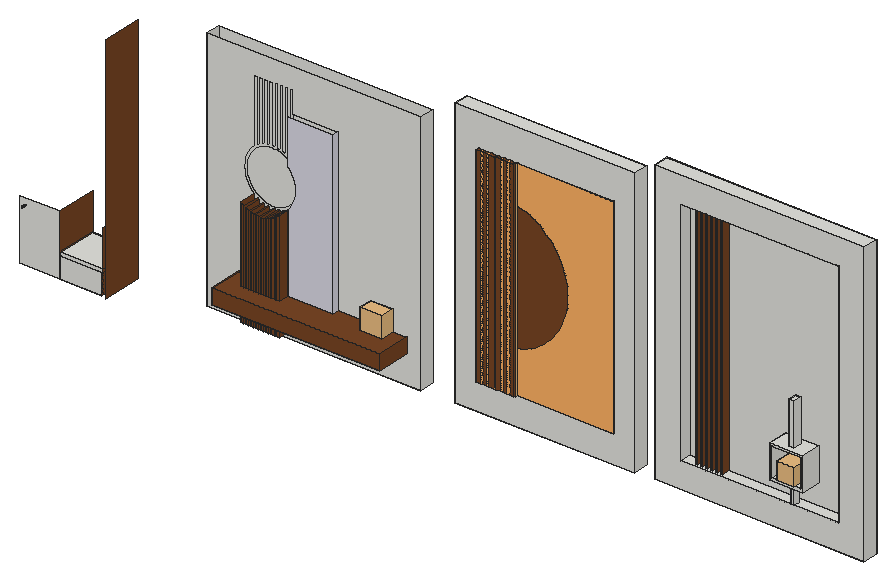
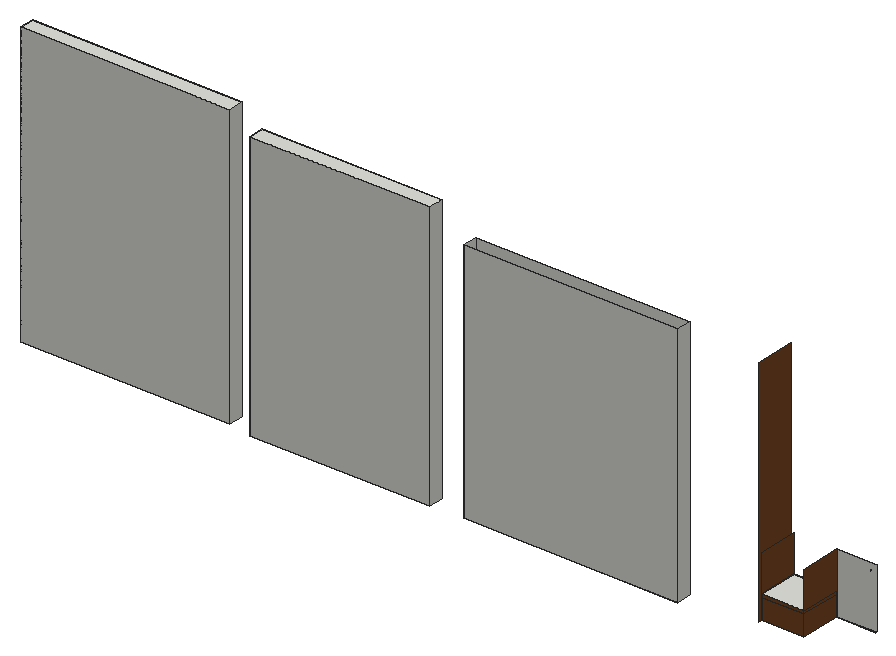
# SketchUp Ruby script. Lengths in inches.
U = 1.inch
M = Sketchup.active_model
def pt(a) = Geom::Point3d.new(a.map { |v| v * U })
def face(e, loops, mat)
  f = e.add_face(loops[0].map { |a| pt(a) })
  loops[1..].each { |l| e.add_face(l.map { |a| pt(a) }).erase! }
  f.material = f.back_material = mat if mat
  f
end
# faces: each face lists its corners as indices into pts; further lists are holes
def faces(e, pts, list, mat = nil) = list.each { |f| face(e, (f[0].is_a?(Array) ? f : [f]).map { |l| l.map { |i| pts[i] } }, mat) }
# xy, xz, yz: faces in a plane at the given z, y or x. An outline is a flat list of corners, or four numbers for a rectangle; further outlines are holes
def ring(l) = l.size == 4 ? [[l[0], l[1]], [l[2], l[1]], [l[2], l[3]], [l[0], l[3]]] : l.each_slice(2).to_a
def flat(e, list, mat, &to3) = list.each { |f| face(e, (f[0].is_a?(Array) ? f : [f]).map { |l| ring(l).map { |u, v| to3.(u, v) } }, mat) }
def xy(e, z, list, mat = nil) = flat(e, list, mat) { |x, y| [x, y, z] }
def xz(e, y, list, mat = nil) = flat(e, list, mat) { |x, z| [x, y, z] }
def yz(e, x, list, mat = nil) = flat(e, list, mat) { |y, z| [x, y, z] }
def lines(e, pts, list) = list.each { |a, b| e.add_line(pt(pts[a]), pt(pts[b])) }
# prism: a flat outline (further loops are holes) pulled along v
def prism(e, loops, v, mat = nil)
  f = face(e, loops, mat); d = Geom::Vector3d.new(v.map { |x| x * U })
  f.pushpull(f.normal.samedirection?(d) ? d.length : -d.length)
end
def box(e, o, s, mat = nil) = prism(e, [[o, [o[0] + s[0], o[1], o[2]], [o[0] + s[0], o[1] + s[1], o[2]], [o[0], o[1] + s[1], o[2]]]], [0, 0, s[2]], mat)
def at(x, y, z, deg = 0) = Geom::Transformation.translation(pt([x, y, z])) * Geom::Transformation.rotation(ORIGIN, Z_AXIS, deg.degrees)
def axes(o, x, y, z) = Geom::Transformation.new([*x, 0, *y, 0, *z, 0, *pt(o).to_a, 1])
def part(name) = M.definitions.add(name)
# library, detail: a bought-in or finely detailed component or shape, given as its bounding box
def library(name, o, s) = part(name).tap { |d| box(d.entities, o, s) }
def detail(e, o, s) = box(e.add_group.entities, o, s)
def put(e, d, t, mat = nil) = e.add_instance(d, t).tap { |i| i.material = mat if mat }
def group(e, t, mat = nil) = e.add_group.tap { |g| g.transformation = t; g.material = mat if mat }.entities
root = M.entities
M.materials.add("[Color A01]").color = [218, 217, 228]
M.materials.add("[Color C03]").color = [255, 178, 101]
M.materials.add("[Wood Veneer 01]").color = [120, 70, 37]
c1 = library("utensil 8",[0,0,0],[7.12,4.41,9.55])
c2 = library("Group\#6",[-0.5,-0.5,0],[1,1.55,124])
c3 = library("Potted fan palm",[0,0,0],[52.56,47.17,54.17])
xy(root,0,[[149.45,26.47,277.45,35.47]])
xy(root,1.59,[[58,2,81.38,2.47],[81.51,2,106.84,2.47],[81.38,2.47,106.84,26.47]],"[Wood Veneer 01]")
xy(root,5.83,[[177.91,16.47,179.91,26.47],[180.91,16.47,182.91,26.47],[183.91,16.47,185.91,26.47],[186.91,16.47,188.91,26.47],[189.91,16.47,191.91,26.47],
  [192.91,16.47,194.91,26.47],[195.91,16.47,197.91,26.47],[198.91,16.47,200.91,26.47]],"[Wood Veneer 01]")
xy(root,8.83,[[200.91,22.47,227.91,26.47]],"[Color A01]")
xy(root,13.59,[[81.51,2,106.84,2.47],[81.38,2.47,106.84,26.47]],"[Wood Veneer 01]")
xy(root,15.59,[[81.38,2.47,106.84,26.47]])
xy(root,16.44,[[168.78,6.47,268.78,26.47]],"[Wood Veneer 01]")
xy(root,16.8125,[[497.84,26.47,499.84,29.73]])
xy(root,25.44,[[168.78,6.47,268.78,26.47]],"[Wood Veneer 01]")
xy(root,28.83,[[[489.27,21.47,509.27,33.47],[497.84,26.47,499.84,29.73]]])
xy(root,30.33,[[490.78,21.47,507.77,33.47]])
xy(root,47.32,[[490.78,21.47,507.77,33.47]])
xy(root,48.83,[[[489.27,21.47,509.27,33.47],[498.36,24.34,501.36,29.34]]])
xy(root,73.83,[[498.36,24.34,501.36,29.34]])
xz(root,0,[[60.68,33.33,60.68,33.34,60.59,33.35,60.59,33.34],[60.68,33.33,60.77,33.34,60.77,33.35,60.68,33.34],[60.59,33.34,60.59,33.35,60.51,33.39,60.5,33.375],[60.68,33.34,60.68,33.35,60.59,33.37,60.59,33.35],[60.68,33.34,60.77,33.35,60.76,33.37,60.68,33.35],
  [60.77,33.34,60.86,33.375,60.85,33.39,60.77,33.35],[60.59,33.35,60.59,33.37,60.51,33.4,60.51,33.39],[60.68,33.35,60.68,33.37,60.6,33.38,60.59,33.37],[60.68,33.35,60.76,33.37,60.76,33.38,60.68,33.37],[60.77,33.35,60.85,33.39,60.84,33.4,60.76,33.37],
  [60.68,33.37,60.76,33.38,60.84,33.41,60.9,33.46,60.95,33.53,60.98,33.6,60.99,33.68,60.98,33.76,60.95,33.84,60.9,33.9,60.84,33.95,60.76,33.99,60.68,34,60.6,33.99,60.52,33.95,60.46,33.9,60.41,33.84,60.375,33.76,60.37,33.68,60.375,33.6,60.41,33.53,60.46,33.46,60.52,33.41,60.6,33.38],[60.59,33.37,60.6,33.38,60.52,33.41,60.51,33.4],[60.76,33.37,60.84,33.4,60.84,33.41,60.76,33.38],[60.5,33.375,60.51,33.39,60.4375,33.44,60.43,33.43],[60.86,33.375,60.93,33.43,60.92,33.44,60.85,33.39],
  [60.51,33.39,60.51,33.4,60.45,33.45,60.4375,33.44],[60.85,33.39,60.92,33.44,60.91,33.45,60.84,33.4],[60.51,33.4,60.52,33.41,60.46,33.46,60.45,33.45],[60.84,33.4,60.91,33.45,60.9,33.46,60.84,33.41],[60.43,33.43,60.4375,33.44,60.38,33.51,60.37,33.5],
  [60.93,33.43,60.99,33.5,60.98,33.51,60.92,33.44],[60.4375,33.44,60.45,33.45,60.39,33.52,60.38,33.51],[60.92,33.44,60.98,33.51,60.96,33.52,60.91,33.45],[60.45,33.45,60.46,33.46,60.41,33.53,60.39,33.52],[60.91,33.45,60.96,33.52,60.95,33.53,60.9,33.46],
  [60.37,33.5,60.38,33.51,60.35,33.59,60.33,33.59],[60.99,33.5,61.02,33.59,61.01,33.59,60.98,33.51],[60.38,33.51,60.39,33.52,60.36,33.6,60.35,33.59],[60.98,33.51,61.01,33.59,61,33.6,60.96,33.52],[60.39,33.52,60.41,33.53,60.375,33.6,60.36,33.6],
  [60.96,33.52,61,33.6,60.98,33.6,60.95,33.53],[60.33,33.59,60.35,33.59,60.34,33.68,60.32,33.68],[60.35,33.59,60.36,33.6,60.35,33.68,60.34,33.68],[61.01,33.59,61.02,33.68,61.01,33.68,61,33.6],[61.01,33.59,61.02,33.59,61.04,33.68,61.02,33.68],
  [60.36,33.6,60.375,33.6,60.37,33.68,60.35,33.68],[60.98,33.6,61,33.6,61.01,33.68,60.99,33.68],[60.32,33.68,60.34,33.68,60.35,33.77,60.33,33.78],[60.34,33.68,60.35,33.68,60.36,33.77,60.35,33.77],[61.01,33.68,61.02,33.68,61.01,33.77,61,33.77],
  [61.02,33.68,61.04,33.68,61.02,33.78,61.01,33.77]],"[Wood Veneer 01]")
xz(root,0.01,[[60.68,33.29,60.68,33.3,60.58,33.3125,60.58,33.3],[60.68,33.29,60.78,33.3,60.78,33.3125,60.68,33.3],[60.58,33.3,60.58,33.3125,60.49,33.35,60.48,33.34],[60.68,33.3,60.68,33.3125,60.58,33.33,60.58,33.3125],[60.68,33.3,60.78,33.3125,60.78,33.33,60.68,33.3125],
  [60.78,33.3,60.875,33.34,60.87,33.35,60.78,33.3125],[60.58,33.3125,60.58,33.33,60.49,33.36,60.49,33.35],[60.78,33.3125,60.87,33.35,60.86,33.36,60.78,33.33],[60.48,33.34,60.49,33.35,60.41,33.41,60.4,33.4],[60.875,33.34,60.96,33.4,60.95,33.41,60.87,33.35],
  [60.49,33.35,60.49,33.36,60.42,33.42,60.41,33.41],[60.87,33.35,60.95,33.41,60.94,33.42,60.86,33.36],[60.4,33.4,60.41,33.41,60.35,33.49,60.34,33.49],[60.96,33.4,61.02,33.49,61.01,33.49,60.95,33.41],[60.41,33.41,60.42,33.42,60.36,33.5,60.35,33.49],
  [60.95,33.41,61.01,33.49,61,33.5,60.94,33.42],[60.34,33.49,60.35,33.49,60.31,33.58,60.3,33.58],[60.35,33.49,60.36,33.5,60.32,33.59,60.31,33.58],[61.01,33.49,61.05,33.58,61.04,33.59,61,33.5],[61.01,33.49,61.02,33.49,61.0625,33.58,61.05,33.58],
  [60.3,33.58,60.31,33.58,60.3,33.68,60.28,33.68],[60.31,33.58,60.32,33.59,60.31,33.68,60.3,33.68],[61.05,33.58,61.0625,33.68,61.05,33.68,61.04,33.59],[61.05,33.58,61.0625,33.58,61.07,33.68,61.0625,33.68]],"[Wood Veneer 01]")
xz(root,0.02,[[60.68,33.27,60.68,33.28,60.57,33.29,60.57,33.28],[60.68,33.27,60.79,33.28,60.78,33.29,60.68,33.28],[60.57,33.28,60.57,33.29,60.48,33.33,60.47,33.32],[60.79,33.28,60.89,33.32,60.88,33.33,60.78,33.29],[60.47,33.32,60.48,33.33,60.39,33.4,60.38,33.39],
  [60.89,33.32,60.97,33.39,60.97,33.4,60.88,33.33],[60.38,33.39,60.39,33.4,60.33,33.48,60.32,33.47],[60.97,33.39,61.04,33.47,61.03,33.48,60.97,33.4],[60.32,33.47,60.33,33.48,60.29,33.58,60.28,33.58],[61.04,33.47,61.08,33.58,61.07,33.58,61.03,33.48],
  [60.28,33.58,60.29,33.58,60.27,33.68,60.26,33.68],[61.07,33.58,61.08,33.58,61.1,33.68,61.09,33.68]],"[Wood Veneer 01]")
xz(root,0.03,[[60.68,33.25,60.68,33.26,60.57,33.27,60.57,33.26],[60.68,33.25,60.79,33.26,60.79,33.27,60.68,33.26],[60.57,33.26,60.57,33.27,60.47,33.3125,60.46,33.31],[60.79,33.26,60.9,33.31,60.89,33.3125,60.79,33.27],[60.46,33.31,60.47,33.3125,60.38,33.38,60.37,33.375],
  [60.9,33.31,60.99,33.375,60.98,33.38,60.89,33.3125],[60.37,33.375,60.38,33.38,60.31,33.47,60.3,33.47],[60.99,33.375,61.06,33.47,61.05,33.47,60.98,33.38],[60.3,33.47,60.31,33.47,60.27,33.57,60.26,33.57],[61.05,33.47,61.06,33.47,61.1,33.57,61.09,33.57],
  [60.26,33.57,60.27,33.57,60.25,33.68,60.24,33.68],[61.09,33.57,61.1,33.57,61.12,33.68,61.11,33.68]],"[Wood Veneer 01]")
xz(root,0.05,[[60.68,33.22,60.68,33.23,60.5625,33.25,60.56,33.24],[60.68,33.22,60.8,33.24,60.8,33.25,60.68,33.23],[60.56,33.24,60.5625,33.25,60.45,33.29,60.45,33.28],[60.8,33.24,60.91,33.28,60.91,33.29,60.8,33.25],[60.45,33.28,60.45,33.29,60.36,33.36,60.35,33.36],
  [60.91,33.28,61.01,33.36,61,33.36,60.91,33.29],[60.35,33.36,60.36,33.36,60.29,33.46,60.28,33.45],[61,33.36,61.01,33.36,61.08,33.45,61.07,33.46],[60.28,33.45,60.29,33.46,60.24,33.57,60.23,33.5625],[61.08,33.45,61.125,33.5625,61.12,33.57,61.07,33.46],
  [61.125,33.5625,61.14,33.68,61.13,33.68,61.12,33.57]],"[Wood Veneer 01]")
xz(root,2,[[[58,1.59,81.38,37.59],[60.68,33.18,60.55,33.2,60.43,33.25,60.33,33.33,60.25,33.43,60.2,33.55,60.18,33.68,60.2,33.8125,60.25,33.93,60.33,34.04,60.43,34.12,60.55,34.17,60.68,34.18,60.81,34.17,60.93,34.12,61.03,34.04,61.11,33.93,61.16,33.8125,61.18,33.68,61.16,33.55,61.11,33.43,61.03,33.33,60.93,33.25,60.81,33.2]],[81.51,1.59,106.84,13.59]])
xz(root,2.47,[[81.38,13.59,106.84,15.59]])
xz(root,2.47,[[81.38,1.59,81.51,13.59]],"[Wood Veneer 01]")
xz(root,6.47,[[168.78,16.44,268.78,25.44]],"[Wood Veneer 01]")
xz(root,16.47,[[177.91,5.83,179.91,5.83,179.91,68.55,179.8,68.61,178.07,69.87,177.91,70.02],[180.91,5.83,182.91,5.83,182.91,67.09,181.67,67.58,180.91,68],[183.91,5.83,185.91,5.83,185.91,66.24,185.72,66.27,183.91,66.73],[186.91,5.83,188.91,5.83,188.91,66,187.84,66,186.91,66.12],[189.91,5.83,191.91,5.83,191.91,66.24,189.98,66,189.91,66],
  [192.91,5.83,194.91,5.83,194.91,67.09,194.16,66.8,192.91,66.48],[195.91,5.83,197.91,5.83,197.91,68.55,196.15,67.58,195.91,67.49],[198.91,5.83,200.91,5.83,200.91,70.96,199.75,69.87,198.91,69.26]],"[Wood Veneer 01]")
xz(root,21.47,[[[489.27,28.83,509.27,48.83],[490.78,30.33,507.77,47.32]]])
xz(root,22.47,[[200.91,8.83,227.91,8.83,227.91,120.83,200.91,120.83,200.91,94.97,201.3,94.6,202.66,92.96,203.81,91.16,204.72,89.22,205.375,87.19,205.78,85.1,205.91,82.97,205.78,80.84,205.375,78.74,204.72,76.71,203.81,74.78,202.66,72.97,201.3,71.33,200.91,70.96]],"[Color A01]")
xz(root,24.34,[[498.36,48.83,501.36,73.83]])
xz(root,26.47,[[[149.45,0,277.45,146],[177.91,5.83,177.91,70.02,176.52,71.33,175.16,72.97,174.01,74.78,173.1,76.71,172.44,78.74,172.04,80.84,171.91,82.97,172.04,85.1,172.44,87.19,173.1,89.22,174.01,91.16,175.16,92.96,176.52,94.6,177.91,95.91,177.91,133.83,179.91,133.83,179.91,97.38,180.91,97.93,180.91,133.83,182.91,133.83,182.91,98.84,183.66,99.13,183.91,99.2,183.91,133.83,185.91,133.83,185.91,99.6875,186.91,99.8125,186.91,133.83,188.91,133.83,188.91,99.93,189.91,99.93,189.91,133.83,191.91,133.83,191.91,99.6875,192.1,99.66,192.91,99.46,192.91,133.83,194.91,133.83,194.91,98.84,195.91,98.44,195.91,133.83,197.91,133.83,197.91,97.38,198.02,97.32,198.91,96.67,198.91,133.83,200.91,133.83,200.91,120.83,227.91,120.83,227.91,8.83,200.91,8.83,200.91,5.83,198.91,5.83,198.91,69.26,198.02,68.61,197.91,68.55,197.91,5.83,195.91,5.83,195.91,67.49,194.91,67.09,194.91,5.83,192.91,5.83,192.91,66.48,192.1,66.27,191.91,66.24,191.91,5.83,189.91,5.83,189.91,66,188.91,66,188.91,5.83,186.91,5.83,186.91,66.12,185.91,66.24,185.91,5.83,183.91,5.83,183.91,66.73,183.66,66.8,182.91,67.09,182.91,5.83,180.91,5.83,180.91,68,179.91,68.55,179.91,5.83]],[177.91,5.83,179.91,5.83,179.91,68.55,180.91,68,180.91,5.83,182.91,5.83,182.91,67.09,183.66,66.8,183.91,66.73,183.91,5.83,185.91,5.83,185.91,66.24,186.91,66.12,186.91,5.83,188.91,5.83,188.91,66,189.91,66,189.91,5.83,191.91,5.83,191.91,66.24,192.1,66.27,192.91,66.48,192.91,5.83,194.91,5.83,194.91,67.09,195.91,67.49,195.91,5.83,197.91,5.83,197.91,68.55,198.02,68.61,198.91,69.26,198.91,5.83,200.91,5.83,200.91,73.03,200.29,72.28,199.96,71.97,198.86,70.9375,198.09,70.38,197.27,69.79,197.24,69.77,195.56,68.84,195.4,68.78,194.4,68.38,193.73,68.12,192.56,67.82,191.83,67.63,191.74,67.62,189.89,67.39,187.93,67.39,187.08,67.49,186.08,67.62,185.98,67.63,184.25,68.08,184.09,68.12,183.42,68.38,182.26,68.84,181.58,69.22,180.58,69.77,180.55,69.79,178.96,70.9375,178.86,71.03,177.53,72.28,176.28,73.79,175.23,75.45,174.4,77.22,173.79,79.08,173.42,81.01,173.3,82.97,173.42,84.92,173.79,86.85,174.4,88.71,175.23,90.49,176.28,92.14,177.53,93.65,178.86,94.9,178.96,94.99,180.55,96.15,180.58,96.16,181.58,96.71,182.26,97.09,183.42,97.55,184.09,97.8125,184.25,97.85,185.98,98.3,187.08,98.4375,187.93,98.54,189.89,98.54,191.74,98.3125,191.83,98.3,192.56,98.11,193.73,97.8125,194.4,97.55,195.4,97.15,195.56,97.09,197.24,96.16,197.27,96.15,198.09,95.55,198.86,94.99,199.96,93.96,200.29,93.65,200.91,92.9,200.91,133.83,198.91,133.83,198.91,96.67,198.02,97.32,197.91,97.38,197.91,133.83,195.91,133.83,195.91,98.44,194.91,98.84,194.91,133.83,192.91,133.83,192.91,99.46,192.1,99.66,191.91,99.6875,191.91,133.83,189.91,133.83,189.91,99.93,188.91,99.93,188.91,133.83,186.91,133.83,186.91,99.8125,185.91,99.6875,185.91,133.83,183.91,133.83,183.91,99.2,183.66,99.13,182.91,98.84,182.91,133.83,180.91,133.83,180.91,97.93,179.91,97.38,179.91,133.83,177.91,133.83,177.91,95.91,176.52,94.6,175.16,92.96,174.01,91.16,173.1,89.22,172.44,87.19,172.04,85.1,171.91,82.97,172.04,80.84,172.44,78.74,173.1,76.71,174.01,74.78,175.16,72.97,176.52,71.33,177.91,70.02],[168.78,16.44,268.78,25.44],[497.84,16.8125,499.84,28.83]])
xz(root,26.47,[[81.38,1.59,106.84,13.59],[81.38,13.59,106.84,15.59]],"[Wood Veneer 01]")
xz(root,29.34,[[498.36,48.83,501.36,73.83]])
xz(root,29.73,[[497.84,16.8125,499.84,28.83]])
xz(root,33.47,[[[489.27,28.83,509.27,48.83],[490.78,30.33,507.77,47.32]],[490.78,30.33,507.77,47.32]])
xz(root,35.47,[[149.45,0,277.45,146]])
yz(root,81.38,[[2,1.59,2.47,13.59],[2.47,1.59,26.47,13.59],[2,13.59,2.47,15.59],[2.47,13.59,26.47,15.59],[2,15.59,26.47,37.59]],"[Wood Veneer 01]")
yz(root,81.51,[[2,1.59,2.47,13.59]],"[Wood Veneer 01]")
yz(root,106.84,[[2,1.59,2.47,13.59],[2.47,1.59,26.47,13.59],[2.47,13.59,26.47,15.59],[2.47,15.59,26.47,37.59]],"[Wood Veneer 01]")
yz(root,108.43,[[2.47,0,26.47,138.34]],"[Wood Veneer 01]")
yz(root,149.45,[[26.47,0,35.47,146]])
yz(root,168.78,[[6.47,16.44,26.47,25.44]],"[Wood Veneer 01]")
yz(root,177.91,[[16.47,5.83,26.47,70.02]],"[Wood Veneer 01]")
yz(root,179.91,[[16.47,5.83,26.47,68.55]],"[Wood Veneer 01]")
yz(root,180.91,[[16.47,5.83,26.47,68]],"[Wood Veneer 01]")
yz(root,182.91,[[16.47,5.83,26.47,67.09]],"[Wood Veneer 01]")
yz(root,183.91,[[16.47,5.83,26.47,66.73]],"[Wood Veneer 01]")
yz(root,185.91,[[16.47,5.83,26.47,66.24]],"[Wood Veneer 01]")
yz(root,186.91,[[16.47,5.83,26.47,66.12]],"[Wood Veneer 01]")
yz(root,188.91,[[16.47,5.83,26.47,66]],"[Wood Veneer 01]")
yz(root,189.91,[[16.47,5.83,26.47,66]],"[Wood Veneer 01]")
yz(root,191.91,[[16.47,5.83,26.47,66.24]],"[Wood Veneer 01]")
yz(root,192.91,[[16.47,5.83,26.47,66.48]],"[Wood Veneer 01]")
yz(root,194.91,[[16.47,5.83,26.47,67.09]],"[Wood Veneer 01]")
yz(root,195.91,[[16.47,5.83,26.47,67.49]],"[Wood Veneer 01]")
yz(root,197.91,[[16.47,5.83,26.47,68.55]],"[Wood Veneer 01]")
yz(root,198.91,[[16.47,5.83,26.47,69.26]],"[Wood Veneer 01]")
yz(root,200.91,[[22.47,8.83,26.47,70.96]])
yz(root,200.91,[[16.47,5.83,26.47,5.83,26.47,8.83,22.47,8.83,22.47,70.96,16.47,70.96]],"[Wood Veneer 01]")
yz(root,227.91,[[22.47,8.83,26.47,120.83]],"[Color A01]")
yz(root,268.78,[[6.47,16.44,26.47,25.44]],"[Wood Veneer 01]")
yz(root,277.45,[[26.47,0,35.47,146]])
yz(root,489.27,[[21.47,28.83,33.47,48.83]])
yz(root,490.78,[[21.47,30.33,33.47,47.32]])
yz(root,497.84,[[26.47,16.8125,29.73,28.83]])
yz(root,498.36,[[24.34,48.83,29.34,73.83]])
yz(root,499.84,[[26.47,16.8125,29.73,28.83]])
yz(root,501.36,[[24.34,48.83,29.34,73.83]])
yz(root,507.77,[[21.47,30.33,33.47,47.32]])
yz(root,509.27,[[21.47,28.83,33.47,48.83]])
p = [[60.45,0.05,33.29],[60.5625,0.05,33.25],[60.5625,0.04,33.25],[60.46,0.04,33.3],[60.68,0.04,33.24],[60.68,0.05,33.23],
  [60.68,0.03,33.25],[60.57,0.03,33.26],[60.79,0.04,33.25],[60.79,0.03,33.26],[60.8,0.05,33.25],[60.9,0.04,33.3],
  [60.91,0.05,33.29],[60.43,0.16,33.25],[60.55,0.16,33.2],[60.55,0.14,33.2],[60.43,0.14,33.25],[60.55,0.13,33.21],
  [60.43,0.13,33.25],[60.55,0.12,33.21],[60.43,0.12,33.26],[60.55,0.1,33.21],[60.44,0.1,33.26],[60.55,0.09,33.22],
  [60.4375,0.09,33.26],[60.56,0.08,33.22],[60.44,0.08,33.27],[60.56,0.07,33.23],[60.44,0.07,33.27],[60.56,0.0625,33.23],
  [60.45,0.0625,33.28],[60.56,0.05,33.24],[60.45,0.05,33.28],[60.68,0.14,33.1875],[60.68,0.16,33.18],[60.68,0.13,33.1875],
  [60.68,0.12,33.19],[60.68,0.1,33.19],[60.68,0.09,33.2],[60.68,0.08,33.2],[60.68,0.07,33.21],[60.68,0.0625,33.22],
  [60.68,0.05,33.22],[60.8,0.0625,33.23],[60.8,0.05,33.24],[60.8,0.07,33.23],[60.8,0.08,33.22],[60.8,0.09,33.22],
  [60.81,0.1,33.21],[60.81,0.12,33.21],[60.81,0.13,33.21],[60.81,0.14,33.2],[60.81,0.16,33.2],[60.91,0.05,33.28],
  [60.91,0.0625,33.28],[60.92,0.07,33.27],[60.92,0.08,33.27],[60.92,0.09,33.26],[60.92,0.1,33.26],[60.93,0.12,33.26],
  [60.93,0.13,33.25],[60.93,0.14,33.25],[60.93,0.16,33.25],[60.43,2,33.25],[60.55,2,33.2],[60.55,0.19,33.2],
  [60.43,0.19,33.25],[60.55,0.17,33.2],[60.43,0.17,33.25],[60.68,2,33.18],[60.68,0.19,33.18],[60.68,0.17,33.18],
  [60.81,0.17,33.2],[60.81,0.19,33.2],[60.81,2,33.2],[60.93,0.17,33.25],[60.93,0.19,33.25],[60.93,2,33.25],
  [60.36,0.04,33.37],[60.36,0.05,33.36],[60.46,0.03,33.31],[60.37,0.03,33.375],[60.47,0.02,33.32],[60.38,0.02,33.39],
  [60.38,0.03,33.38],[60.47,0.03,33.3125],[60.48,0.01,33.34],[60.4,0.01,33.4],[60.39,0.02,33.4],[60.48,0.02,33.33],
  [60.57,0.03,33.27],[60.57,0.02,33.28],[60.57,0.02,33.29],[60.58,0.01,33.3],[60.49,0.01,33.36],[60.58,0.01,33.33],
  [60.59,0,33.34],[60.5,0,33.375],[60.68,0.02,33.27],[60.68,0.03,33.26],[60.68,0.01,33.29],[60.68,0.02,33.28],
  [60.68,0,33.33],[60.68,0.01,33.3125],[60.78,0.01,33.33],[60.77,0,33.34],[60.78,0.02,33.29],[60.78,0.01,33.3],
  [60.79,0.03,33.27],[60.79,0.02,33.28],[60.86,0,33.375],[60.86,0.01,33.36],[60.875,0.01,33.34],[60.88,0.02,33.33],
  [60.89,0.02,33.32],[60.89,0.03,33.3125],[60.9,0.03,33.31],[60.97,0.02,33.4],[60.96,0.01,33.4],[60.98,0.03,33.38],
  [60.97,0.02,33.39],[60.99,0.04,33.37],[60.99,0.03,33.375],[61,0.05,33.36],[60.25,0.16,33.43],[60.33,0.16,33.33],
  [60.33,0.14,33.33],[60.25,0.14,33.43],[60.33,0.13,33.33],[60.25,0.13,33.4375],[60.33,0.12,33.34],[60.25,0.12,33.4375],
  [60.33,0.1,33.34],[60.26,0.1,33.4375],[60.34,0.09,33.34],[60.26,0.09,33.44],[60.34,0.08,33.34],[60.26,0.08,33.44],
  [60.34,0.07,33.35],[60.27,0.07,33.45],[60.35,0.0625,33.35],[60.27,0.0625,33.45],[60.35,0.05,33.36],[61.01,0.0625,33.35],
  [61.01,0.05,33.36],[61.01,0.07,33.35],[61.02,0.08,33.34],[61.02,0.09,33.34],[61.02,0.1,33.34],[61.03,0.12,33.34],
  [61.03,0.13,33.33],[61.03,0.14,33.33],[61.03,0.16,33.33],[61.09,0.07,33.45],[61.08,0.0625,33.45],[61.09,0.08,33.44],
  [61.1,0.09,33.44],[61.1,0.1,33.4375],[61.11,0.12,33.4375],[61.11,0.13,33.4375],[61.11,0.14,33.43],[61.11,0.16,33.43],
  [60.25,2,33.43],[60.33,2,33.33],[60.33,0.19,33.33],[60.25,0.19,33.43],[60.33,0.17,33.33],[60.25,0.17,33.43],
  [61.03,0.17,33.33],[61.03,0.19,33.33],[61.03,2,33.33],[61.11,0.17,33.43],[61.11,0.19,33.43],[61.11,2,33.43],
  [60.29,0.05,33.46],[60.29,0.04,33.46],[60.3,0.03,33.47],[60.31,0.03,33.47],[60.32,0.02,33.47],[60.33,0.02,33.48],
  [60.34,0.01,33.49],[60.36,0.01,33.5],[60.42,0.01,33.42],[60.43,0,33.43],[60.37,0,33.5],[60.94,0.01,33.42],
  [60.93,0,33.43],[61,0.01,33.5],[60.99,0,33.5],[61.03,0.02,33.48],[61.02,0.01,33.49],[61.05,0.03,33.47],
  [61.04,0.02,33.47],[61.06,0.04,33.46],[61.06,0.03,33.47],[61.07,0.05,33.46],[60.22,0.07,33.5625],[60.22,0.08,33.56],
  [60.23,0.0625,33.5625],[60.28,0.05,33.45],[60.23,0.05,33.5625],[61.08,0.05,33.45],[61.125,0.05,33.5625],[61.13,0.0625,33.5625],
  [61.14,0.07,33.5625],[61.14,0.08,33.56],[61.15,0.09,33.56],[61.15,0.1,33.56],[61.15,0.12,33.56],[61.16,0.13,33.56],
  [61.16,0.14,33.55],[61.16,0.16,33.55],[61.16,0.17,33.55],[61.16,0.19,33.55],[61.16,2,33.55],[60.25,0.04,33.57],
  [60.24,0.05,33.57],[60.26,0.03,33.57],[60.28,0.02,33.58],[60.27,0.03,33.57],[60.3,0.01,33.58],[60.29,0.02,33.58],
  [60.33,0,33.59],[60.32,0.01,33.59],[61.02,0,33.59],[61.04,0.01,33.59],[61.0625,0.01,33.58],[61.07,0.02,33.58],
  [61.08,0.02,33.58],[61.09,0.03,33.57],[61.1,0.03,33.57],[61.11,0.04,33.57],[61.12,0.05,33.57],[60.24,0.03,33.68],
  [60.23,0.04,33.68],[60.26,0.02,33.68],[60.25,0.03,33.68],[60.28,0.01,33.68],[60.27,0.02,33.68],[60.32,0,33.68],
  [60.31,0.01,33.68],[61.05,0.01,33.68],[61.04,0,33.68],[61.09,0.02,33.68],[61.07,0.01,33.68],[61.11,0.03,33.68],
  [61.1,0.02,33.68],[61.125,0.04,33.68],[61.12,0.03,33.68],[61.13,0.05,33.68],[61.15,0.0625,33.68],[61.14,0.05,33.68],
  [61.15,0.07,33.68],[61.16,0.08,33.68],[61.16,0.09,33.68],[61.17,0.1,33.68],[61.17,0.12,33.68],[61.17,0.13,33.68],
  [61.18,0.14,33.68],[61.18,0.16,33.68],[61.18,0.17,33.68],[61.18,0.19,33.68],[61.18,2,33.68]]
faces(root,p,[[0,1,2,3],[4,2,1,5],[6,7,2,4],[4,8,9,6],[5,10,8,4],[11,8,10,12],[13,14,15,16],[16,15,17,18],
  [18,17,19,20],[20,19,21,22],[22,21,23,24],[24,23,25,26],[26,25,27,28],[28,27,29,30],[30,29,31,32],[33,15,14,34],
  [35,17,15,33],[36,19,17,35],[37,21,19,36],[38,23,21,37],[39,25,23,38],[40,27,25,39],[41,29,27,40],[42,31,29,41],
  [41,43,44,42],[40,45,43,41],[39,46,45,40],[38,47,46,39],[37,48,47,38],[36,49,48,37],[35,50,49,36],[33,51,50,35],
  [34,52,51,33],[53,44,43,54],[54,43,45,55],[55,45,46,56],[56,46,47,57],[57,47,48,58],[58,48,49,59],[59,49,50,60],
  [60,50,51,61],[61,51,52,62],[63,64,65,66],[66,65,67,68],[68,67,14,13],[64,69,70,65],[71,67,65,70],[34,14,67,71],
  [71,72,52,34],[70,73,72,71],[69,74,73,70],[62,52,72,75],[75,72,73,76],[74,77,76,73],[3,78,79,0],[80,81,78,3],
  [82,83,84,85],[86,87,88,89],[3,2,7,80],[85,90,91,82],[89,92,93,86],[94,95,96,97],[98,91,90,99],[100,93,92,101],
  [102,96,95,103],[103,104,105,102],[101,106,107,100],[99,108,109,98],[110,105,104,111],[112,107,106,113],[114,109,108,115],[116,9,8,11],
  [113,117,118,112],[115,119,120,114],[11,121,122,116],[12,123,121,11],[124,125,126,127],[127,126,128,129],[129,128,130,131],[131,130,132,133],
  [133,132,134,135],[135,134,136,137],[137,136,138,139],[139,138,140,141],[16,126,125,13],[18,128,126,16],[20,130,128,18],[22,132,130,20],
  [24,134,132,22],[26,136,134,24],[28,138,136,26],[30,140,138,28],[32,142,140,30],[54,143,144,53],[55,145,143,54],[56,146,145,55],
  [57,147,146,56],[58,148,147,57],[59,149,148,58],[60,150,149,59],[61,151,150,60],[62,152,151,61],[145,153,154,143],[146,155,153,145],
  [147,156,155,146],[148,157,156,147],[149,158,157,148],[150,159,158,149],[151,160,159,150],[152,161,160,151],[162,163,164,165],[165,164,166,167],
  [167,166,125,124],[163,63,66,164],[68,166,164,66],[13,125,166,68],[75,168,152,62],[76,169,168,75],[77,170,169,76],[168,171,161,152],
  [169,172,171,168],[170,173,172,169],[174,79,78,175],[175,78,81,176],[177,84,83,178],[179,88,87,180],[181,182,183,184],[97,183,182,94],
  [111,185,186,110],[185,187,188,186],[117,189,190,118],[119,191,192,120],[121,193,194,122],[123,195,193,121],[139,196,197,137],[141,198,196,139],
  [199,200,198,141],[141,140,142,199],[143,154,201,144],[202,201,154,203],[203,154,153,204],[204,153,155,205],[205,155,156,206],[206,156,157,207],
  [207,157,158,208],[208,158,159,209],[209,159,160,210],[210,160,161,211],[211,161,171,212],[212,171,172,213],[173,214,213,172],[175,215,216,174],
  [176,217,215,175],[178,218,219,177],[180,220,221,179],[184,222,223,181],[224,188,187,225],[226,190,189,227],[228,192,191,229],[230,194,193,231],
  [231,193,195,232],[217,233,234,215],[218,235,236,219],[220,237,238,221],[222,239,240,223],[225,241,242,224],[227,243,244,226],[229,245,246,228],
  [231,247,248,230],[232,249,247,231],[203,250,251,202],[204,252,250,203],[205,253,252,204],[206,254,253,205],[207,255,254,206],[208,256,255,207],
  [209,257,256,208],[210,258,257,209],[211,259,258,210],[212,260,259,211],[213,261,260,212],[214,262,261,213]],"[Wood Veneer 01]")
put(root,c1,axes([247.79,18.05,25.44],[1.8318,0,0],[0,1.81,0],[0,0,1.29]))
put(root,c2,at(333.68,26.43,16.88))
g1 = group(root,at(296.93,25.47,0))
g2 = group(g1,at(13.91,0,16.88),"[Color C03]")
xy(g2,0,[[0,0,2.75,2],[2.75,0,4,2],[4,0,6.75,2],[6.75,0,8,2],[8,0,10.75,2],
  [10.75,0,12,2],[12,0,14.75,2],[14.75,0,16,2],[16,0,18.75,2],[18.75,0,20,2],
  [20,0,22.75,2],[22.75,1.5,81,2]])
xy(g2,124,[[2.75,0,4,2],[6.75,0,8,2],[10.75,0,12,2],[14.75,0,16,2],[18.75,0,20,2],
  [22.75,1.5,81,2]])
xy(g2,124,[[0,0,2.75,2],[4,0,6.75,2],[8,0,10.75,2],[12,0,14.75,2],[16,0,18.75,2],
  [20,0,22.75,2]],"[Wood Veneer 01]")
xz(g2,0,[[2.75,0,4,124],[6.75,0,8,124],[10.75,0,12,124],[14.75,0,16,124],[18.75,0,20,124]])
xz(g2,0,[[0,0,2.75,124],[4,0,6.75,124],[8,0,10.75,124],[12,0,14.75,124],[16,0,18.75,124],
  [20,0,22.75,124]],"[Wood Veneer 01]")
xz(g2,1.5,[[22.75,0,81,0,81,124,22.75,124,22.75,101.83,25.34,101.18,27.88,100.35,30.36,99.34,32.76,98.18,35.08,96.85,37.3,95.37,39.42,93.74,41.42,91.97,43.3,90.07,45.04,88.05,46.64,85.91,48.1,83.67,49.4,81.34,50.54,78.92,51.51,76.4375,52.3125,73.89,52.94,71.29,53.39,68.66,53.66,66,53.75,63.33,53.66,60.67,53.39,58.01,52.94,55.375,52.3125,52.78,51.51,50.23,50.54,47.74,49.4,45.33,48.1,43,46.64,40.76,45.04,38.62,43.3,36.6,41.42,34.7,39.42,32.93,37.3,31.3,35.08,29.82,32.76,28.49,30.36,27.33,27.88,26.32,25.34,25.49,22.75,24.83]])
xz(g2,1.5,[[22.75,24.83,25.34,25.49,27.88,26.32,30.36,27.33,32.76,28.49,35.08,29.82,37.3,31.3,39.42,32.93,41.42,34.7,43.3,36.6,45.04,38.62,46.64,40.76,48.1,43,49.4,45.33,50.54,47.74,51.51,50.23,52.3125,52.78,52.94,55.375,53.39,58.01,53.66,60.67,53.75,63.33,53.66,66,53.39,68.66,52.94,71.29,52.3125,73.89,51.51,76.4375,50.54,78.92,49.4,81.34,48.1,83.67,46.64,85.91,45.04,88.05,43.3,90.07,41.42,91.97,39.42,93.74,37.3,95.37,35.08,96.85,32.76,98.18,30.36,99.34,27.88,100.35,25.34,101.18,22.75,101.83]],"[Wood Veneer 01]")
yz(g2,0,[[0,0,2,124]],"[Wood Veneer 01]")
yz(g2,22.75,[[0.95,0,1.5,124]])
yz(g2,22.75,[[0,0,0.95,124]],"[Wood Veneer 01]")
yz(g2,81,[[1.5,0,2,124]])
g3 = group(g1,at(0,2,0))
box(g3,[0,0,0],[107,9,160])
g4 = group(root,at(439.53,28.47,16.8125),"[Wood Veneer 01]")
box(g4,[3,0,0],[1.02,5,137.29])
box(g4,[9,0,0],[1.02,5,137.29])
box(g4,[12,0,0],[1.02,5,137.29])
box(g4,[15,0,0],[1.02,5,137.29])
box(g4,[6,0,0],[1.02,5,137.29])
box(g4,[0,0,0],[1.02,5,137.29])
g5 = group(root,at(416.69,26.47,1.46))
xy(g5,0,[[0,0,125,9]])
xy(g5,15.36,[[15.36,0,109.64,7]])
xy(g5,152.64,[[15.36,0,109.64,7]])
xy(g5,168,[[0,0,125,9]])
xz(g5,0,[[[0,0,125,168],[15.36,15.36,109.64,152.64]]])
xz(g5,7,[[15.36,15.36,109.64,152.64]])
xz(g5,9,[[0,0,125,168]])
yz(g5,0,[[0,0,9,168]])
yz(g5,15.36,[[0,15.36,7,152.64]])
yz(g5,109.64,[[0,15.36,7,152.64]])
yz(g5,125,[[0,0,9,168]])
put(root,c3,axes([494.05,20.72,30.85],[0.19673,0,0],[0,0.20632,0],[0,0,0.18864]))
